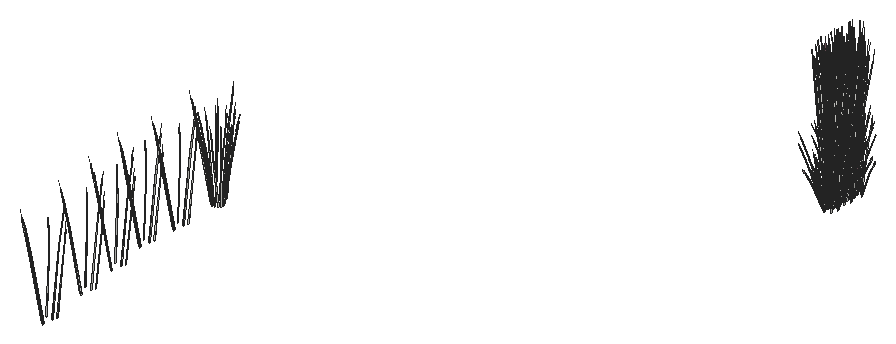
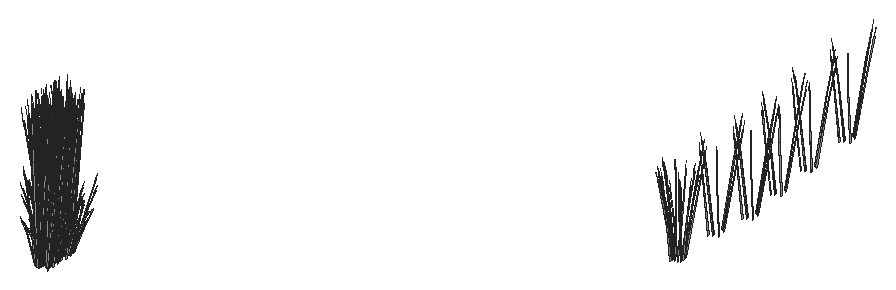
# SketchUp Ruby script. Lengths in inches.
U = 1.inch
M = Sketchup.active_model
def pt(a) = Geom::Point3d.new(a.map { |v| v * U })
def face(e, loops, mat)
  f = e.add_face(loops[0].map { |a| pt(a) })
  loops[1..].each { |l| e.add_face(l.map { |a| pt(a) }).erase! }
  f.material = f.back_material = mat if mat
  f
end
# faces: each face lists its corners as indices into pts; further lists are holes
def faces(e, pts, list, mat = nil) = list.each { |f| face(e, (f[0].is_a?(Array) ? f : [f]).map { |l| l.map { |i| pts[i] } }, mat) }
# xy, xz, yz: faces in a plane at the given z, y or x. An outline is a flat list of corners, or four numbers for a rectangle; further outlines are holes
def ring(l) = l.size == 4 ? [[l[0], l[1]], [l[2], l[1]], [l[2], l[3]], [l[0], l[3]]] : l.each_slice(2).to_a
def flat(e, list, mat, &to3) = list.each { |f| face(e, (f[0].is_a?(Array) ? f : [f]).map { |l| ring(l).map { |u, v| to3.(u, v) } }, mat) }
def xy(e, z, list, mat = nil) = flat(e, list, mat) { |x, y| [x, y, z] }
def xz(e, y, list, mat = nil) = flat(e, list, mat) { |x, z| [x, y, z] }
def yz(e, x, list, mat = nil) = flat(e, list, mat) { |y, z| [x, y, z] }
def lines(e, pts, list) = list.each { |a, b| e.add_line(pt(pts[a]), pt(pts[b])) }
# prism: a flat outline (further loops are holes) pulled along v
def prism(e, loops, v, mat = nil)
  f = face(e, loops, mat); d = Geom::Vector3d.new(v.map { |x| x * U })
  f.pushpull(f.normal.samedirection?(d) ? d.length : -d.length)
end
def box(e, o, s, mat = nil) = prism(e, [[o, [o[0] + s[0], o[1], o[2]], [o[0] + s[0], o[1] + s[1], o[2]], [o[0], o[1] + s[1], o[2]]]], [0, 0, s[2]], mat)
def at(x, y, z, deg = 0) = Geom::Transformation.translation(pt([x, y, z])) * Geom::Transformation.rotation(ORIGIN, Z_AXIS, deg.degrees)
def axes(o, x, y, z) = Geom::Transformation.new([*x, 0, *y, 0, *z, 0, *pt(o).to_a, 1])
def part(name) = M.definitions.add(name)
# library, detail: a bought-in or finely detailed component or shape, given as its bounding box
def library(name, o, s) = part(name).tap { |d| box(d.entities, o, s) }
def detail(e, o, s) = box(e.add_group.entities, o, s)
def put(e, d, t, mat = nil) = e.add_instance(d, t).tap { |i| i.material = mat if mat }
def group(e, t, mat = nil) = e.add_group.tap { |g| g.transformation = t; g.material = mat if mat }.entities
root = M.entities
M.materials.add("LightPink_Translucent").color = [144, 107, 117]
M.materials["LightPink_Translucent"].alpha = 0.75
c1 = part("blade")
p = [[2.15,0.21,22],[0,0.17,0],[0.09,0.45,0],[2.18,0.31,22],[2.29,0.31,22],[0.38,0.45,0],
  [2.48,0.24,33],[2.49,0.24,33],[2.48,0.22,33]]
faces(c1.entities,p,[[0,1,2,3],[4,5,2,3],[6,3,4,7],[8,0,3,6]])
c2 = part("seeds")
p = [[0.3,-0.1,1.38],[-0.01,-0.03,1.59],[-0.01,-0.03,0.03],[0.14,-0.07,-0.07],[0.29,-0.03,3],[0.15,0.01,3.11]]
faces(c2.entities,p,[[0,1,2,3],[1,0,4,5]],"LightPink_Translucent")
c3 = part("blade with seeds")
put(c3.entities,c1,at(0,0,0))
put(c3.entities,c2,axes([2.4,0.25,30.99],[1.5799,-0.05474,1.17369],[-0.12525,1.92788,0.29478],[-0.07173,-0.02425,1.56792]))
put(root,c3,axes([301.4,192.37,151.3],[0.45651,-0.12123,0.45419],[0.07923,0.47555,0.3745],[-0.10736,-0.14016,0.93983]))
put(root,c3,axes([300.48,193.0625,151.3],[0.33843,-0.34808,0.45419],[0.29188,0.36965,0.3745],[-0.15878,-0.06421,0.93983]))
put(root,c3,axes([299.71,196.17,151.77],[0.36162,0.1259,-0.05481],[-0.11124,0.3875,-0.2485],[-0.05915,0.05883,0.81966]))
put(root,c3,axes([302.26,197.55,151.77],[0.28319,-0.27058,-0.05481],[0.25948,0.29635,-0.2485],[0.01827,0.08397,0.81966]))
put(root,c3,axes([301.77,196.55,151.28],[-0.4038,-0.12331,0.45013],[0.13808,-0.40538,0.37115],[0.02427,0.15942,0.93144]))
put(root,c3,axes([299.4,211.78,151.3],[0.45651,-0.12123,0.45419],[0.07923,0.47555,0.3745],[-0.10736,-0.14016,0.93983]))
put(root,c3,axes([298.48,212.47,151.3],[0.33843,-0.34808,0.45419],[0.29188,0.36965,0.3745],[-0.15878,-0.06421,0.93983]))
put(root,c3,axes([297.71,215.58,151.77],[0.36162,0.1259,-0.05481],[-0.11124,0.3875,-0.2485],[-0.05915,0.05883,0.81966]))
put(root,c3,axes([300.26,216.96,151.77],[0.28319,-0.27058,-0.05481],[0.25948,0.29635,-0.2485],[0.01827,0.08397,0.81966]))
put(root,c3,axes([299.77,215.96,151.28],[-0.4038,-0.12331,0.45013],[0.13808,-0.40538,0.37115],[0.02427,0.15942,0.93144]))
put(root,c3,axes([297.5,227.38,151.3],[0.45651,-0.12123,0.45419],[0.07923,0.47555,0.3745],[-0.10736,-0.14016,0.93983]))
put(root,c3,axes([296.58,228.07,151.3],[0.33843,-0.34808,0.45419],[0.29188,0.36965,0.3745],[-0.15878,-0.06421,0.93983]))
put(root,c3,axes([295.81,231.18,151.77],[0.36162,0.1259,-0.05481],[-0.11124,0.3875,-0.2485],[-0.05915,0.05883,0.81966]))
put(root,c3,axes([298.36,232.56,151.77],[0.28319,-0.27058,-0.05481],[0.25948,0.29635,-0.2485],[0.01827,0.08397,0.81966]))
put(root,c3,axes([297.87,231.5625,151.28],[-0.4038,-0.12331,0.45013],[0.13808,-0.40538,0.37115],[0.02427,0.15942,0.93144]))
put(root,c3,axes([295.27,242.54,151.3],[0.45651,-0.12123,0.45419],[0.07923,0.47555,0.3745],[-0.10736,-0.14016,0.93983]))
put(root,c3,axes([294.35,243.24,151.3],[0.33843,-0.34808,0.45419],[0.29188,0.36965,0.3745],[-0.15878,-0.06421,0.93983]))
put(root,c3,axes([293.57,246.34,151.77],[0.36162,0.1259,-0.05481],[-0.11124,0.3875,-0.2485],[-0.05915,0.05883,0.81966]))
put(root,c3,axes([296.13,247.72,151.77],[0.28319,-0.27058,-0.05481],[0.25948,0.29635,-0.2485],[0.01827,0.08397,0.81966]))
put(root,c3,axes([295.64,246.72,151.28],[-0.4038,-0.12331,0.45013],[0.13808,-0.40538,0.37115],[0.02427,0.15942,0.93144]))
put(root,c3,axes([296.74,255.59,151.3],[0.45651,-0.12123,0.45419],[0.07923,0.47555,0.3745],[-0.10736,-0.14016,0.93983]))
put(root,c3,axes([295.82,256.28,151.3],[0.33843,-0.34808,0.45419],[0.29188,0.36965,0.3745],[-0.15878,-0.06421,0.93983]))
put(root,c3,axes([295.05,259.39,151.77],[0.36162,0.1259,-0.05481],[-0.11124,0.3875,-0.2485],[-0.05915,0.05883,0.81966]))
put(root,c3,axes([297.6,260.77,151.77],[0.28319,-0.27058,-0.05481],[0.25948,0.29635,-0.2485],[0.01827,0.08397,0.81966]))
put(root,c3,axes([297.11,259.77,151.28],[-0.4038,-0.12331,0.45013],[0.13808,-0.40538,0.37115],[0.02427,0.15942,0.93144]))
put(root,c3,axes([296.03,273.2,151.3],[0.45651,-0.12123,0.45419],[0.07923,0.47555,0.3745],[-0.10736,-0.14016,0.93983]))
put(root,c3,axes([297.06,273.58,151.27],[-0.12355,0.36271,0.29918],[-0.36044,-0.10579,-0.38624],[-0.03305,-0.14603,0.73904]))
put(root,c3,axes([297.83,273.99,151.27],[-0.27728,0.24833,0.29918],[-0.26248,-0.28355,-0.38624],[0.03994,-0.14407,0.73904]))
put(root,c3,axes([296.19,273.64,151.27],[0.06329,0.37991,0.29918],[-0.36182,0.10032,-0.38624],[-0.09718,-0.10887,0.73904]))
put(root,c3,axes([295.1,273.89,151.3],[0.33843,-0.34808,0.45419],[0.29188,0.36965,0.3745],[-0.15878,-0.06421,0.93983]))
put(root,c3,axes([298.31,274.76,151.27],[-0.35672,0.06741,0.29918],[-0.09419,-0.38534,-0.38624],[0.10222,-0.1035,0.73904]))
put(root,c3,axes([295.47,274.16,151.27],[0.23317,0.29531,0.29918],[-0.26625,0.27955,-0.38624],[-0.13527,-0.04253,0.73904]))
put(root,c3,axes([298.37,275.68,151.27],[-0.34057,-0.13158,0.29918],[0.09933,-0.38387,-0.38624],[0.13712,-0.0352,0.73904]))
put(root,c3,axes([295.09,274.98,151.27],[0.34057,0.13158,0.29918],[-0.09933,0.38387,-0.38624],[-0.13712,0.0352,0.73904]))
put(root,c3,axes([297.99,276.51,151.27],[-0.23317,-0.29531,0.29918],[0.26625,-0.27955,-0.38624],[0.13527,0.04253,0.73904]))
put(root,c3,axes([295.14,275.91,151.27],[0.35672,-0.06741,0.29918],[0.09419,0.38534,-0.38624],[-0.10222,0.1035,0.73904]))
put(root,c3,axes([294.33,277,151.77],[0.36162,0.1259,-0.05481],[-0.11124,0.3875,-0.2485],[-0.05915,0.05883,0.81966]))
put(root,c3,axes([297.27,277.02,151.27],[-0.06329,-0.37991,0.29918],[0.36182,-0.10032,-0.38624],[0.09718,0.10887,0.73904]))
put(root,c3,axes([295.625,276.67,151.27],[0.27728,-0.24833,0.29918],[0.26248,0.28355,-0.38624],[-0.03994,0.14407,0.73904]))
put(root,c3,axes([296.4,277.08,151.27],[0.12355,-0.36271,0.29918],[0.36044,0.10579,-0.38624],[0.03305,0.14603,0.73904]))
put(root,c3,axes([296.89,278.375,151.77],[0.28319,-0.27058,-0.05481],[0.25948,0.29635,-0.2485],[0.01827,0.08397,0.81966]))
put(root,c3,axes([296.4,277.38,151.28],[-0.4038,-0.12331,0.45013],[0.13808,-0.40538,0.37115],[0.02427,0.15942,0.93144]))
put(root,c3,axes([429.88,376.04,152.1875],[-0.11649,0.09547,1.20808],[-0.34886,-0.1671,-0.25981],[0.06467,-0.20781,0.51652]))
put(root,c3,axes([428.08,375.86,152.1875],[-0.02482,0.15429,1.20808],[-0.36278,0.12916,-0.25981],[-0.0848,-0.19943,0.51652]))
put(root,c3,axes([429.02,375.52,151.26],[-0.06874,0.01699,1.48974],[-0.38012,-0.19128,-0.22758],[0.00638,-0.15955,0.25375]))
put(root,c3,axes([429.46,375.28,152.34],[0.05257,0.27504,0.97034],[-0.29163,-0.15233,0.71294],[0.03138,-0.14083,0.21373]))
put(root,c3,axes([427.96,375.61,152.34],[0.21377,0.16416,0.97034],[-0.31132,0.09868,0.71294],[-0.06661,-0.12616,0.21373]))
put(root,c3,axes([427.79,376.11,151.26],[-0.0397,0.06213,1.48974],[-0.40116,0.13396,-0.22758],[-0.09691,-0.12186,0.25375]))
put(root,c3,axes([430.7,376.34,151.26],[-0.06134,-0.03716,1.48974],[-0.15755,-0.41512,-0.22758],[0.10629,-0.11265,0.25375]))
put(root,c3,axes([428.38,376.42,152],[-0.25622,-0.47263,0],[0.42866,-0.26357,-0.43598],[0.09763,-0.06003,1.38303]))
put(root,c3,axes([428.95,375.86,151.8],[-0.28319,0.27058,-0.03288],[-0.25948,-0.29635,-0.1491],[-0.01827,-0.08397,0.4918]))
put(root,c3,axes([431.01,377.17,152.1875],[-0.1464,-0.01397,1.20808],[-0.14998,-0.37477,-0.25981],[0.17985,-0.10602,0.51652]))
put(root,c3,axes([431.18,376.48,152.34],[-0.1365,0.2401,0.97034],[-0.11733,-0.32258,0.71294],[0.11274,-0.08083,0.21373]))
put(root,c3,axes([428.89,377.73,152.25],[-0.04775,-0.53819,-0.2458],[0.49736,-0.03254,-0.42242],[0.08758,-0.07169,1.34921]))
put(root,c3,axes([427.54,376.35,151.8],[-0.11822,0.38513,-0.03288],[-0.36385,-0.11847,-0.1491],[-0.05524,-0.06299,0.4918]))
put(root,c3,axes([428.66,378.29,152.25],[-0.46151,-0.22505,-0.2458],[0.22222,-0.475,-0.42242],[-0.0145,-0.11662,1.34921]))
put(root,c3,axes([427.34,378.11,152],[-0.51243,0,0],[0,-0.52715,-0.43598],[0,-0.12006,1.38303]))
put(root,c3,axes([427.43,377.16,152.1875],[0.08001,0.13132,1.20808],[-0.18437,0.35694,-0.25981],[-0.18931,-0.08532,0.51652]))
put(root,c3,axes([427.74,377.97,151.97],[-0.38118,0.39654,0.25983],[-0.38142,-0.39237,-0.30828],[-0.01331,-0.11261,1.39295]))
put(root,c3,axes([428.95,378.15,152.06],[0.46174,0.2286,0.2033],[-0.22222,0.475,0.42242],[0,-0.1095,1.35626]))
put(root,c3,axes([428.77,378.79,152.06],[0.10862,-0.55889,-0.19793],[0.515,0.09742,0.43313],[-0.08999,-0.07718,1.32161]))
put(root,c3,axes([426.95,377.56,152.34],[0.26163,-0.03375,0.97034],[-0.16596,0.29737,0.71294],[-0.12929,-0.04461,0.21373]))
put(root,c3,axes([428.8,377.83,152.3],[-0.44501,0.02912,0.37796],[-0.04024,-0.48332,-0.1819],[0.07967,-0.04899,1.2135]))
put(root,c3,axes([427.65,378.19,152.09],[0,0.47166,0.41945],[-0.45849,0,0],[0,-0.10742,1.33059]))
put(root,c3,axes([430.27,376.54,152.01],[0.25622,-0.47263,0],[0.42866,0.26357,-0.43598],[0.09763,0.06003,1.38303]))
put(root,c3,axes([428.79,378.01,151.99],[0.17817,0.52741,0.38653],[-0.50909,0.1834,0.15168],[0.00622,-0.09691,1.34202]))
put(root,c3,axes([431.28,378.41,151.67],[-0.26394,0.0566,1.1961],[-0.04201,-0.45055,0.06846],[0.18486,-0.06819,0.68062]))
put(root,c3,axes([431.76,378.01,151.91],[-0.25407,-0.3016,-0.05481],[0.27826,-0.27635,-0.2485],[0.07884,-0.01946,0.81966]))
put(root,c3,axes([428.7,378.42,152.3],[-0.19883,0.425,0.37796],[-0.41314,-0.20454,-0.1819],[0,-0.09797,1.2135]))
put(root,c3,axes([429.43,378.05,151.86],[0,-0.54574,0],[0.51243,0,0],[0,0,1.51605]))
put(root,c3,axes([430.05,376.79,152.09],[-0.38354,-0.23583,0.41945],[0.22925,-0.42288,0],[0.08735,0.05371,1.33059]))
put(root,c3,axes([429.18,377.71,151.99],[-0.33979,0.42804,0.38653],[-0.40368,-0.37784,0.15168],[0.08192,-0.04272,1.34202]))
put(root,c3,axes([429.56,378.47,151.94],[-0.38118,-0.40596,-0.0518],[0.38142,-0.40621,0],[-0.01331,-0.01418,1.48322]))
put(root,c3,axes([428.59,377,152.09],[-0.11838,0.46875,0.14904],[-0.43321,-0.13265,0.29641],[0.07483,-0.00228,1.35512]))
put(root,c3,axes([428.42,377.38,151.35],[-0.40337,0.18883,1.08919],[-0.12839,-0.54182,0.42321],[0.24769,0.00901,1.23883]))
put(root,c3,axes([429.5,377.52,152.21],[0.07906,-0.42093,0.12232],[0.38625,0.07307,-0.3493],[0.07029,0.04322,1.07074]))
put(root,c3,axes([428.83,378.52,151.99],[0.51796,0.09937,0.38653],[-0.10541,0.56124,0.15168],[-0.07569,-0.05419,1.34202]))
put(root,c3,axes([431.57,378.12,151.26],[-0.02142,-0.07161,1.48974],[0.14855,-0.41887,-0.22758],[0.14984,-0.00603,0.25375]))
put(root,c3,axes([427.14,378.04,151.26],[0.01039,0.07433,1.48974],[-0.20952,0.38819,-0.22758],[-0.14882,-0.01957,0.25375]))
put(root,c3,axes([429.33,377.63,152.3],[-0.24618,-0.39589,0.37796],[0.37289,-0.27878,-0.1819],[0.07967,0.04899,1.2135]))
put(root,c3,axes([428.55,379.42,152.09],[0.44036,-0.12519,0.14904],[0.10874,0.46588,0.29641],[-0.03927,-0.06788,1.35512]))
put(root,c3,axes([429.46,377.66,152.25],[0.41376,-0.31314,-0.2458],[0.27514,0.44246,-0.42242],[0.10209,0.04493,1.34921]))
put(root,c3,axes([429.88,381.79,152.1875],[-0.11649,0.09547,1.20808],[-0.34886,-0.1671,-0.25981],[0.06467,-0.20781,0.51652]))
put(root,c3,axes([428.08,381.61,152.1875],[-0.02482,0.15429,1.20808],[-0.36278,0.12916,-0.25981],[-0.0848,-0.19943,0.51652]))
put(root,c3,axes([429.78,378.17,151.86],[0.45849,0,0],[0,0.4883,0],[0,0,1.50718]))
put(root,c3,axes([429,378.79,152.25],[-0.41376,0.31314,-0.2458],[-0.27514,-0.44246,-0.42242],[-0.10209,-0.04493,1.34921]))
put(root,c3,axes([429.91,377.03,152.09],[-0.44036,0.12519,0.14904],[-0.10874,-0.46588,0.29641],[0.03927,0.06788,1.35512]))
put(root,c3,axes([429.02,381.27,151.26],[-0.06874,0.01699,1.48974],[-0.38012,-0.19128,-0.22758],[0.00638,-0.15955,0.25375]))
put(root,c3,axes([429.63,377.92,152.01],[-0.51796,-0.09937,0.41563],[0.10541,-0.56124,0.1631],[0.07569,0.05419,1.44303]))
put(root,c3,axes([429.21,379.3125,151.86],[-0.13371,-0.40664,0],[0.38182,-0.1424,0],[0,0,1.30413]))
put(root,c3,axes([428.96,378.92,152.21],[-0.07906,0.42093,0.12232],[-0.38625,-0.07307,-0.3493],[-0.07029,-0.04322,1.07074]))
put(root,c3,axes([429.71,379.25,151.85],[0.43024,-0.16003,-0.16218],[0.15118,0.46099,0.00007],[0.04749,-0.01769,1.46908]))
put(root,c3,axes([429.86,379.45,152.09],[0.11838,-0.46875,0.14904],[0.43321,0.13265,0.29641],[-0.07483,0.00228,1.35512]))
put(root,c3,axes([429.46,381.03,152.34],[0.05257,0.27504,0.97034],[-0.29163,-0.15233,0.71294],[0.03138,-0.14083,0.21373]))
put(root,c3,axes([429.77,378.38,151.87],[0.28606,0.30466,0],[-0.28606,0.30466,0],[0,0,1.42996]))
put(root,c3,axes([430.54,378.25,152.09],[-0.32198,-0.34356,0.14904],[0.32447,-0.33323,0.29641],[-0.03556,0.07016,1.35512]))
put(root,c3,axes([431.83,378.5625,152.34],[-0.2532,0.07787,0.97034],[0.11918,-0.32181,0.71294],[0.13432,0.02202,0.21373]))
put(root,c3,axes([429.12,379.49,151.86],[-0.41314,-0.21175,0],[0.19883,-0.43999,0],[0,0,1.37455]))
put(root,c3,axes([429.46,378.93,152.08],[-0.40016,-0.37963,-0.21282],[0.33672,-0.42629,0.46574],[-0.10776,0.04441,1.42109]))
put(root,c3,axes([428.41,379.66,152.09],[0.38354,0.23583,0.41945],[-0.22925,0.42288,0],[-0.08735,-0.05371,1.33059]))
put(root,c3,axes([429.76,378.03,152.3],[0.19883,-0.425,0.37796],[0.41314,0.20454,-0.1819],[0,0.09797,1.2135]))
put(root,c3,axes([427.96,381.36,152.34],[0.21377,0.16416,0.97034],[-0.31132,0.09868,0.71294],[-0.06661,-0.12616,0.21373]))
put(root,c3,axes([429.68,378.27,151.9375],[0,0.54548,-0.04762],[-0.51243,0,0],[0,0.01714,1.5153]))
put(root,c3,axes([428.1875,379.91,152],[-0.25622,0.47263,0],[-0.42866,-0.26357,-0.43598],[-0.09763,-0.06003,1.38303]))
put(root,c3,axes([430.8,378.26,152.09],[0,-0.47166,0.41945],[0.45849,0,0],[0,0.10742,1.33059]))
put(root,c3,axes([429.66,378.62,152.3],[0.44501,-0.02912,0.37796],[0.04024,0.48332,-0.1819],[-0.07967,0.04899,1.2135]))
put(root,c3,axes([429.93,378.125,152.21],[0.38182,-0.13755,0.12232],[0.13371,0.39278,-0.3493],[0,0.08644,1.07074]))
put(root,c3,axes([427.79,381.86,151.26],[-0.0397,0.06213,1.48974],[-0.40116,0.13396,-0.22758],[-0.09691,-0.12186,0.25375]))
put(root,c3,axes([431.35,379.08,152.1875],[-0.0987,-0.116,1.20808],[0.12841,-0.38374,-0.25981],[0.19968,0.05198,0.51652]))
put(root,c3,axes([429.59,379.5,151.86],[0.41314,0.21175,0],[-0.19883,0.43999,0],[0,0,1.47801]))
put(root,c3,axes([430.7,382.08,151.26],[-0.06134,-0.03716,1.48974],[-0.15755,-0.41512,-0.22758],[0.10629,-0.11265,0.25375]))
put(root,c3,axes([429.75,379.97,151.85],[-0.25302,-0.47428,-0.04344],[0.42866,-0.26357,0.43598],[-0.10563,0.04516,1.38235]))
put(root,c3,axes([429.66,378.82,152.21],[0.30276,0.28338,0.12232],[-0.25254,0.31972,-0.3493],[-0.07029,0.04322,1.07074]))
put(root,c3,axes([428.38,382.17,152],[-0.25622,-0.47263,0],[0.42866,-0.26357,-0.43598],[0.09763,-0.06003,1.38303]))
put(root,c3,axes([428.95,381.6,151.8],[-0.28319,0.27058,-0.03288],[-0.25948,-0.29635,-0.1491],[-0.01827,-0.08397,0.4918]))
put(root,c3,axes([429.99,379.7,152.09],[0.38354,-0.23583,0.41945],[0.22925,0.42288,0],[-0.08735,0.05371,1.33059]))
put(root,c3,axes([429.44,379.32,151.9375],[0.17817,0.54185,-0.05079],[-0.50909,0.18987,0],[0.00622,0.01892,1.45452]))
put(root,c3,axes([426.88,379.08,152.1875],[0.14242,0.03872,1.20808],[0.09179,0.39548,-0.25981],[-0.19345,0.07403,0.51652]))
put(root,c3,axes([431.12,378.34,152.01],[0.51243,0,0],[0,0.52715,-0.43598],[0,0.12006,1.38303]))
put(root,c3,axes([430.91,378.61,151.86],[-0.51218,-0.00377,-0.04204],[0,-0.52715,0.42192],[-0.0161,0.12,1.33776]))
put(root,c3,axes([429.8,378.16,152.25],[0.46151,0.22505,-0.2458],[-0.22222,0.475,-0.42242],[0.0145,0.11662,1.34921]))
put(root,c3,axes([426.58,379.91,152.34],[0.17079,-0.21377,0.97034],[0.06739,0.33841,0.71294],[-0.12342,0.0606,0.21373]))
put(root,c3,axes([429.57,378.72,152.25],[0.04775,0.53819,-0.2458],[-0.49736,0.03254,-0.42242],[-0.08758,0.07169,1.34921]))
put(root,c3,axes([431.01,382.91,152.1875],[-0.1464,-0.01397,1.20808],[-0.14998,-0.37477,-0.25981],[0.17985,-0.10602,0.51652]))
put(root,c3,axes([431.18,382.23,152.34],[-0.1365,0.2401,0.97034],[-0.11733,-0.32258,0.71294],[0.11274,-0.08083,0.21373]))
put(root,c3,axes([429.76,379.73,151.97],[0.51304,0.1533,0.25983],[-0.12835,0.54797,-0.30828],[-0.08491,0.06858,1.39295]))
put(root,c3,axes([428.89,383.48,152.25],[-0.04775,-0.53819,-0.2458],[0.49736,-0.03254,-0.42242],[0.08758,-0.07169,1.34921]))
put(root,c3,axes([427.54,382.09,151.8],[-0.11822,0.38513,-0.03288],[-0.36385,-0.11847,-0.1491],[-0.05524,-0.06299,0.4918]))
put(root,c3,axes([428.66,384.04,152.25],[-0.46151,-0.22505,-0.2458],[0.22222,-0.475,-0.42242],[-0.0145,-0.11662,1.34921]))
put(root,c3,axes([430.42,379.68,152.34],[-0.23074,-0.13562,0.97034],[0.29794,-0.1378,0.71294],[0.08036,0.11673,0.21373]))
put(root,c3,axes([427.34,383.85,152],[-0.51243,0,0],[0,-0.52715,-0.43598],[0,-0.12006,1.38303]))
put(root,c3,axes([427.43,382.91,152.1875],[0.08001,0.13132,1.20808],[-0.18437,0.35694,-0.25981],[-0.18931,-0.08532,0.51652]))
put(root,c3,axes([430.08,380.02,152],[0.25622,0.47263,0],[-0.42866,0.26357,-0.43598],[-0.09763,0.06003,1.38303]))
put(root,c3,axes([430.48,380.18,151.26],[0.02986,-0.06809,1.48974],[0.37589,-0.20055,-0.22758],[0.11396,0.1038,0.25375]))
put(root,c3,axes([429.86,378.15,152.4],[-0.01119,-0.44408,1.19347],[0.50665,0.11511,0.50532],[-0.11983,0.243,1.12654]))
put(root,c3,axes([427.03,380.125,151.26],[0.05497,0.04712,1.48974],[0.09321,0.43661,-0.22758],[-0.12183,0.0931,0.25375]))
put(root,c3,axes([427.74,383.71,151.97],[-0.38118,0.39654,0.25983],[-0.38142,-0.39237,-0.30828],[-0.01331,-0.11261,1.39295]))
put(root,c3,axes([430.46,380.3,152.25],[-0.26279,-0.01479,0.88755],[0.17355,-0.31417,0.49003],[0.10382,0.11162,0.6962]))
put(root,c3,axes([428.95,383.9,152.06],[0.46174,0.2286,0.2033],[-0.22222,0.475,0.42242],[0,-0.1095,1.35626]))
put(root,c3,axes([428.77,384.54,152.06],[0.10862,-0.55889,-0.19793],[0.515,0.09742,0.43313],[-0.08999,-0.07718,1.32161]))
put(root,c3,axes([426.95,383.31,152.34],[0.26163,-0.03375,0.97034],[-0.16596,0.29737,0.71294],[-0.12929,-0.04461,0.21373]))
put(root,c3,axes([428.8,383.58,152.3],[-0.44501,0.02912,0.37796],[-0.04024,-0.48332,-0.1819],[0.07967,-0.04899,1.2135]))
put(root,c3,axes([429.6,379.53,152.1875],[0.00723,-0.15635,1.20808],[0.34559,-0.17464,-0.25981],[0.10668,0.18713,0.51652]))
put(root,c3,axes([427.65,383.93,152.09],[0,0.47166,0.41945],[-0.45849,0,0],[0,-0.10742,1.33059]))
put(root,c3,axes([429.88,386.36,152.1875],[-0.11649,0.09547,1.20808],[-0.34886,-0.1671,-0.25981],[0.06467,-0.20781,0.51652]))
put(root,c3,axes([430.27,382.29,152.01],[0.25622,-0.47263,0],[0.42866,0.26357,-0.43598],[0.09763,0.06003,1.38303]))
put(root,c3,axes([428.79,383.75,151.99],[0.17817,0.52741,0.38653],[-0.50909,0.1834,0.15168],[0.00622,-0.09691,1.34202]))
put(root,c3,axes([428.08,386.18,152.1875],[-0.02482,0.15429,1.20808],[-0.36278,0.12916,-0.25981],[-0.0848,-0.19943,0.51652]))
put(root,c3,axes([428.03,380.84,152.34],[-0.01061,-0.28045,0.97034],[0.26501,0.20003,0.71294],[-0.05212,0.13367,0.21373]))
put(root,c3,axes([431.28,384.16,151.67],[-0.26394,0.0566,1.1961],[-0.04201,-0.45055,0.06846],[0.18486,-0.06819,0.68062]))
put(root,c3,axes([431.76,383.76,151.91],[-0.25407,-0.3016,-0.05481],[0.27826,-0.27635,-0.2485],[0.07884,-0.01946,0.81966]))
put(root,c3,axes([429.02,385.84,151.26],[-0.06874,0.01699,1.48974],[-0.38012,-0.19128,-0.22758],[0.00638,-0.15955,0.25375]))
put(root,c3,axes([428.7,384.17,152.3],[-0.19883,0.425,0.37796],[-0.41314,-0.20454,-0.1819],[0,-0.09797,1.2135]))
put(root,c3,axes([429.43,383.8,151.86],[0,-0.54574,0],[0.51243,0,0],[0,0,1.51605]))
put(root,c3,axes([428.73,380.17,151.26],[0.06632,-0.02567,1.48974],[0.39894,0.14126,-0.22758],[0.01167,0.15921,0.25375]))
put(root,c3,axes([430.05,382.54,152.09],[-0.38354,-0.23583,0.41945],[0.22925,-0.42288,0],[0.08735,0.05371,1.33059]))
put(root,c3,axes([429.18,383.46,151.99],[-0.33979,0.42804,0.38653],[-0.40368,-0.37784,0.15168],[0.08192,-0.04272,1.34202]))
put(root,c3,axes([427.8125,380.23,152.38],[0.37228,-0.08352,0.05498],[0.08559,0.3365,-0.7291],[-0.0236,0.17034,0.65354]))
put(root,c3,axes([429.56,384.22,151.94],[-0.38118,-0.40596,-0.0518],[0.38142,-0.40621,0],[-0.01331,-0.01418,1.48322]))
put(root,c3,axes([428.59,382.75,152.09],[-0.11838,0.46875,0.14904],[-0.43321,-0.13265,0.29641],[0.07483,-0.00228,1.35512]))
put(root,c3,axes([429.46,385.6,152.34],[0.05257,0.27504,0.97034],[-0.29163,-0.15233,0.71294],[0.03138,-0.14083,0.21373]))
put(root,c3,axes([428.42,383.13,151.35],[-0.40337,0.18883,1.08919],[-0.12839,-0.54182,0.42321],[0.24769,0.00901,1.23883]))
put(root,c3,axes([429.5,383.27,152.21],[0.07906,-0.42093,0.12232],[0.38625,0.07307,-0.3493],[0.07029,0.04322,1.07074]))
put(root,c3,axes([428.83,384.27,151.99],[0.51796,0.09937,0.38653],[-0.10541,0.56124,0.15168],[-0.07569,-0.05419,1.34202]))
put(root,c3,axes([431.57,383.86,151.26],[-0.02142,-0.07161,1.48974],[0.14855,-0.41887,-0.22758],[0.14984,-0.00603,0.25375]))
put(root,c3,axes([427.14,383.79,151.26],[0.01039,0.07433,1.48974],[-0.20952,0.38819,-0.22758],[-0.14882,-0.01957,0.25375]))
put(root,c3,axes([429.33,383.38,152.3],[-0.24618,-0.39589,0.37796],[0.37289,-0.27878,-0.1819],[0.07967,0.04899,1.2135]))
put(root,c3,axes([428.55,385.17,152.09],[0.44036,-0.12519,0.14904],[0.10874,0.46588,0.29641],[-0.03927,-0.06788,1.35512]))
put(root,c3,axes([429.46,383.41,152.25],[0.41376,-0.31314,-0.2458],[0.27514,0.44246,-0.42242],[0.10209,0.04493,1.34921]))
put(root,c3,axes([427.96,385.93,152.34],[0.21377,0.16416,0.97034],[-0.31132,0.09868,0.71294],[-0.06661,-0.12616,0.21373]))
put(root,c3,axes([429.78,383.92,151.86],[0.45849,0,0],[0,0.4883,0],[0,0,1.50718]))
put(root,c3,axes([427.72,380.59,152.1875],[0.12932,-0.07441,1.20808],[0.31929,0.22435,-0.25981],[-0.09503,0.19413,0.51652]))
put(root,c3,axes([429,384.54,152.25],[-0.41376,0.31314,-0.2458],[-0.27514,-0.44246,-0.42242],[-0.10209,-0.04493,1.34921]))
put(root,c3,axes([429.91,382.78,152.09],[-0.44036,0.12519,0.14904],[-0.10874,-0.46588,0.29641],[0.03927,0.06788,1.35512]))
put(root,c3,axes([427.79,386.43,151.26],[-0.0397,0.06213,1.48974],[-0.40116,0.13396,-0.22758],[-0.09691,-0.12186,0.25375]))
put(root,c3,axes([429.63,383.67,152.01],[-0.51796,-0.09937,0.41563],[0.10541,-0.56124,0.1631],[0.07569,0.05419,1.44303]))
put(root,c3,axes([429.21,385.06,151.86],[-0.13371,-0.40664,0],[0.38182,-0.1424,0],[0,0,1.30413]))
put(root,c3,axes([430.7,386.66,151.26],[-0.06134,-0.03716,1.48974],[-0.15755,-0.41512,-0.22758],[0.10629,-0.11265,0.25375]))
put(root,c3,axes([428.96,384.67,152.21],[-0.07906,0.42093,0.12232],[-0.38625,-0.07307,-0.3493],[-0.07029,-0.04322,1.07074]))
put(root,c3,axes([429.71,385,151.85],[0.43024,-0.16003,-0.16218],[0.15118,0.46099,0.00007],[0.04749,-0.01769,1.46908]))
put(root,c3,axes([429.86,385.19,152.09],[0.11838,-0.46875,0.14904],[0.43321,0.13265,0.29641],[-0.07483,0.00228,1.35512]))
put(root,c3,axes([429.77,384.13,151.87],[0.28606,0.30466,0],[-0.28606,0.30466,0],[0,0,1.42996]))
put(root,c3,axes([430.54,384,152.09],[-0.32198,-0.34356,0.14904],[0.32447,-0.33323,0.29641],[-0.03556,0.07016,1.35512]))
put(root,c3,axes([431.83,384.3125,152.34],[-0.2532,0.07787,0.97034],[0.11918,-0.32181,0.71294],[0.13432,0.02202,0.21373]))
put(root,c3,axes([429.12,385.24,151.86],[-0.41314,-0.21175,0],[0.19883,-0.43999,0],[0,0,1.37455]))
put(root,c3,axes([429.46,384.68,152.08],[-0.40016,-0.37963,-0.21282],[0.33672,-0.42629,0.46574],[-0.10776,0.04441,1.42109]))
put(root,c3,axes([428.41,385.41,152.09],[0.38354,0.23583,0.41945],[-0.22925,0.42288,0],[-0.08735,-0.05371,1.33059]))
put(root,c3,axes([428.38,386.74,152],[-0.25622,-0.47263,0],[0.42866,-0.26357,-0.43598],[0.09763,-0.06003,1.38303]))
put(root,c3,axes([429.76,383.77,152.3],[0.19883,-0.425,0.37796],[0.41314,0.20454,-0.1819],[0,0.09797,1.2135]))
put(root,c3,axes([428.95,386.17,151.8],[-0.28319,0.27058,-0.03288],[-0.25948,-0.29635,-0.1491],[-0.01827,-0.08397,0.4918]))
put(root,c3,axes([429.68,384.02,151.9375],[0,0.54548,-0.04762],[-0.51243,0,0],[0,0.01714,1.5153]))
put(root,c3,axes([428.1875,385.65,152],[-0.25622,0.47263,0],[-0.42866,-0.26357,-0.43598],[-0.09763,-0.06003,1.38303]))
put(root,c3,axes([430.8,384.01,152.09],[0,-0.47166,0.41945],[0.45849,0,0],[0,0.10742,1.33059]))
put(root,c3,axes([429.66,384.36,152.3],[0.44501,-0.02912,0.37796],[0.04024,0.48332,-0.1819],[-0.07967,0.04899,1.2135]))
put(root,c3,axes([429.93,383.87,152.21],[0.38182,-0.13755,0.12232],[0.13371,0.39278,-0.3493],[0,0.08644,1.07074]))
put(root,c3,axes([431.01,387.48,152.1875],[-0.1464,-0.01397,1.20808],[-0.14998,-0.37477,-0.25981],[0.17985,-0.10602,0.51652]))
put(root,c3,axes([431.35,384.83,152.1875],[-0.0987,-0.116,1.20808],[0.12841,-0.38374,-0.25981],[0.19968,0.05198,0.51652]))
put(root,c3,axes([431.18,386.8,152.34],[-0.1365,0.2401,0.97034],[-0.11733,-0.32258,0.71294],[0.11274,-0.08083,0.21373]))
put(root,c3,axes([429.59,385.25,151.86],[0.41314,0.21175,0],[-0.19883,0.43999,0],[0,0,1.47801]))
put(root,c3,axes([429.75,385.72,151.85],[-0.25302,-0.47428,-0.04344],[0.42866,-0.26357,0.43598],[-0.10563,0.04516,1.38235]))
put(root,c3,axes([429.66,384.57,152.21],[0.30276,0.28338,0.12232],[-0.25254,0.31972,-0.3493],[-0.07029,0.04322,1.07074]))
put(root,c3,axes([428.89,388.05,152.25],[-0.04775,-0.53819,-0.2458],[0.49736,-0.03254,-0.42242],[0.08758,-0.07169,1.34921]))
put(root,c3,axes([427.54,386.67,151.8],[-0.11822,0.38513,-0.03288],[-0.36385,-0.11847,-0.1491],[-0.05524,-0.06299,0.4918]))
put(root,c3,axes([428.66,388.61,152.25],[-0.46151,-0.22505,-0.2458],[0.22222,-0.475,-0.42242],[-0.0145,-0.11662,1.34921]))
put(root,c3,axes([427.34,388.42,152],[-0.51243,0,0],[0,-0.52715,-0.43598],[0,-0.12006,1.38303]))
put(root,c3,axes([429.99,385.44,152.09],[0.38354,-0.23583,0.41945],[0.22925,0.42288,0],[-0.08735,0.05371,1.33059]))
put(root,c3,axes([427.43,387.48,152.1875],[0.08001,0.13132,1.20808],[-0.18437,0.35694,-0.25981],[-0.18931,-0.08532,0.51652]))
put(root,c3,axes([429.44,385.07,151.9375],[0.17817,0.54185,-0.05079],[-0.50909,0.18987,0],[0.00622,0.01892,1.45452]))
put(root,c3,axes([426.88,384.83,152.1875],[0.14242,0.03872,1.20808],[0.09179,0.39548,-0.25981],[-0.19345,0.07403,0.51652]))
put(root,c3,axes([431.12,384.09,152.01],[0.51243,0,0],[0,0.52715,-0.43598],[0,0.12006,1.38303]))
put(root,c3,axes([430.91,384.36,151.86],[-0.51218,-0.00377,-0.04204],[0,-0.52715,0.42192],[-0.0161,0.12,1.33776]))
put(root,c3,axes([429.8,383.9,152.25],[0.46151,0.22505,-0.2458],[-0.22222,0.475,-0.42242],[0.0145,0.11662,1.34921]))
put(root,c3,axes([426.58,385.65,152.34],[0.17079,-0.21377,0.97034],[0.06739,0.33841,0.71294],[-0.12342,0.0606,0.21373]))
put(root,c3,axes([429.57,384.47,152.25],[0.04775,0.53819,-0.2458],[-0.49736,0.03254,-0.42242],[-0.08758,0.07169,1.34921]))
put(root,c3,axes([427.74,388.28,151.97],[-0.38118,0.39654,0.25983],[-0.38142,-0.39237,-0.30828],[-0.01331,-0.11261,1.39295]))
put(root,c3,axes([428.95,388.47,152.06],[0.46174,0.2286,0.2033],[-0.22222,0.475,0.42242],[0,-0.1095,1.35626]))
put(root,c3,axes([428.77,389.11,152.06],[0.10862,-0.55889,-0.19793],[0.515,0.09742,0.43313],[-0.08999,-0.07718,1.32161]))
put(root,c3,axes([429.76,385.48,151.97],[0.51304,0.1533,0.25983],[-0.12835,0.54797,-0.30828],[-0.08491,0.06858,1.39295]))
put(root,c3,axes([426.95,387.875,152.34],[0.26163,-0.03375,0.97034],[-0.16596,0.29737,0.71294],[-0.12929,-0.04461,0.21373]))
put(root,c3,axes([428.8,388.15,152.3],[-0.44501,0.02912,0.37796],[-0.04024,-0.48332,-0.1819],[0.07967,-0.04899,1.2135]))
put(root,c3,axes([427.65,388.5,152.09],[0,0.47166,0.41945],[-0.45849,0,0],[0,-0.10742,1.33059]))
put(root,c3,axes([430.42,385.43,152.34],[-0.23074,-0.13562,0.97034],[0.29794,-0.1378,0.71294],[0.08036,0.11673,0.21373]))
put(root,c3,axes([430.27,386.86,152.01],[0.25622,-0.47263,0],[0.42866,0.26357,-0.43598],[0.09763,0.06003,1.38303]))
put(root,c3,axes([428.79,388.33,151.99],[0.17817,0.52741,0.38653],[-0.50909,0.1834,0.15168],[0.00622,-0.09691,1.34202]))
put(root,c3,axes([431.28,388.73,151.67],[-0.26394,0.0566,1.1961],[-0.04201,-0.45055,0.06846],[0.18486,-0.06819,0.68062]))
put(root,c3,axes([431.76,388.33,151.91],[-0.25407,-0.3016,-0.05481],[0.27826,-0.27635,-0.2485],[0.07884,-0.01946,0.81966]))
put(root,c3,axes([428.7,388.74,152.3],[-0.19883,0.425,0.37796],[-0.41314,-0.20454,-0.1819],[0,-0.09797,1.2135]))
put(root,c3,axes([429.43,388.37,151.86],[0,-0.54574,0],[0.51243,0,0],[0,0,1.51605]))
put(root,c3,axes([430.08,385.77,152],[0.25622,0.47263,0],[-0.42866,0.26357,-0.43598],[-0.09763,0.06003,1.38303]))
put(root,c3,axes([430.05,387.11,152.09],[-0.38354,-0.23583,0.41945],[0.22925,-0.42288,0],[0.08735,0.05371,1.33059]))
put(root,c3,axes([430.48,385.93,151.26],[0.02986,-0.06809,1.48974],[0.37589,-0.20055,-0.22758],[0.11396,0.1038,0.25375]))
put(root,c3,axes([429.86,383.9,152.4],[-0.01119,-0.44408,1.19347],[0.50665,0.11511,0.50532],[-0.11983,0.243,1.12654]))
put(root,c3,axes([427.03,385.875,151.26],[0.05497,0.04712,1.48974],[0.09321,0.43661,-0.22758],[-0.12183,0.0931,0.25375]))
put(root,c3,axes([429.18,388.03,151.99],[-0.33979,0.42804,0.38653],[-0.40368,-0.37784,0.15168],[0.08192,-0.04272,1.34202]))
put(root,c3,axes([429.56,388.79,151.94],[-0.38118,-0.40596,-0.0518],[0.38142,-0.40621,0],[-0.01331,-0.01418,1.48322]))
put(root,c3,axes([428.59,387.32,152.09],[-0.11838,0.46875,0.14904],[-0.43321,-0.13265,0.29641],[0.07483,-0.00228,1.35512]))
put(root,c3,axes([430.46,386.04,152.25],[-0.26279,-0.01479,0.88755],[0.17355,-0.31417,0.49003],[0.10382,0.11162,0.6962]))
put(root,c3,axes([428.42,387.7,151.35],[-0.40337,0.18883,1.08919],[-0.12839,-0.54182,0.42321],[0.24769,0.00901,1.23883]))
put(root,c3,axes([429.5,387.84,152.21],[0.07906,-0.42093,0.12232],[0.38625,0.07307,-0.3493],[0.07029,0.04322,1.07074]))
put(root,c3,axes([428.83,388.84,151.99],[0.51796,0.09937,0.38653],[-0.10541,0.56124,0.15168],[-0.07569,-0.05419,1.34202]))
put(root,c3,axes([431.57,388.4375,151.26],[-0.02142,-0.07161,1.48974],[0.14855,-0.41887,-0.22758],[0.14984,-0.00603,0.25375]))
put(root,c3,axes([427.14,388.36,151.26],[0.01039,0.07433,1.48974],[-0.20952,0.38819,-0.22758],[-0.14882,-0.01957,0.25375]))
put(root,c3,axes([429.33,387.95,152.3],[-0.24618,-0.39589,0.37796],[0.37289,-0.27878,-0.1819],[0.07967,0.04899,1.2135]))
put(root,c3,axes([429.6,385.28,152.1875],[0.00723,-0.15635,1.20808],[0.34559,-0.17464,-0.25981],[0.10668,0.18713,0.51652]))
put(root,c3,axes([428.55,389.74,152.09],[0.44036,-0.12519,0.14904],[0.10874,0.46588,0.29641],[-0.03927,-0.06788,1.35512]))
put(root,c3,axes([429.46,387.98,152.25],[0.41376,-0.31314,-0.2458],[0.27514,0.44246,-0.42242],[0.10209,0.04493,1.34921]))
put(root,c3,axes([429.78,388.49,151.86],[0.45849,0,0],[0,0.4883,0],[0,0,1.50718]))
put(root,c3,axes([428.03,386.59,152.34],[-0.01061,-0.28045,0.97034],[0.26501,0.20003,0.71294],[-0.05212,0.13367,0.21373]))
put(root,c3,axes([429,389.11,152.25],[-0.41376,0.31314,-0.2458],[-0.27514,-0.44246,-0.42242],[-0.10209,-0.04493,1.34921]))
put(root,c3,axes([429.91,387.35,152.09],[-0.44036,0.12519,0.14904],[-0.10874,-0.46588,0.29641],[0.03927,0.06788,1.35512]))
put(root,c3,axes([428.73,385.92,151.26],[0.06632,-0.02567,1.48974],[0.39894,0.14126,-0.22758],[0.01167,0.15921,0.25375]))
put(root,c3,axes([429.63,388.24,152.01],[-0.51796,-0.09937,0.41563],[0.10541,-0.56124,0.1631],[0.07569,0.05419,1.44303]))
put(root,c3,axes([429.21,389.63,151.86],[-0.13371,-0.40664,0],[0.38182,-0.1424,0],[0,0,1.30413]))
put(root,c3,axes([427.8125,385.98,152.38],[0.37228,-0.08352,0.05498],[0.08559,0.3365,-0.7291],[-0.0236,0.17034,0.65354]))
put(root,c3,axes([428.96,389.24,152.21],[-0.07906,0.42093,0.12232],[-0.38625,-0.07307,-0.3493],[-0.07029,-0.04322,1.07074]))
put(root,c3,axes([429.71,389.57,151.85],[0.43024,-0.16003,-0.16218],[0.15118,0.46099,0.00007],[0.04749,-0.01769,1.46908]))
put(root,c3,axes([429.86,389.76,152.09],[0.11838,-0.46875,0.14904],[0.43321,0.13265,0.29641],[-0.07483,0.00228,1.35512]))
put(root,c3,axes([429.77,388.7,151.87],[0.28606,0.30466,0],[-0.28606,0.30466,0],[0,0,1.42996]))
